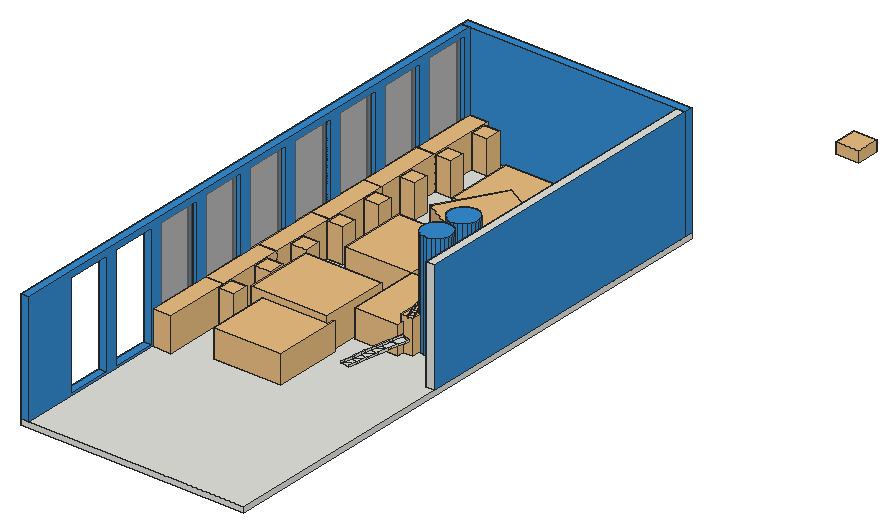
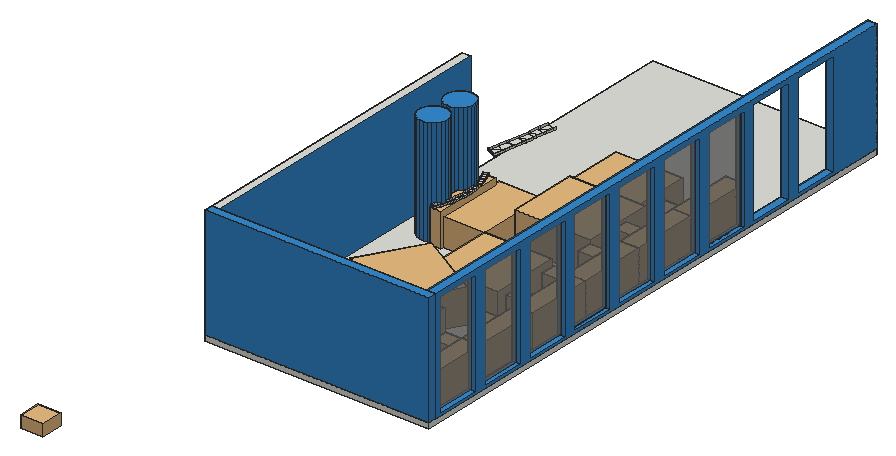
# SketchUp Ruby script. Lengths in inches.
U = 1.inch
M = Sketchup.active_model
def pt(a) = Geom::Point3d.new(a.map { |v| v * U })
def face(e, loops, mat)
  f = e.add_face(loops[0].map { |a| pt(a) })
  loops[1..].each { |l| e.add_face(l.map { |a| pt(a) }).erase! }
  f.material = f.back_material = mat if mat
  f
end
# faces: each face lists its corners as indices into pts; further lists are holes
def faces(e, pts, list, mat = nil) = list.each { |f| face(e, (f[0].is_a?(Array) ? f : [f]).map { |l| l.map { |i| pts[i] } }, mat) }
# xy, xz, yz: faces in a plane at the given z, y or x. An outline is a flat list of corners, or four numbers for a rectangle; further outlines are holes
def ring(l) = l.size == 4 ? [[l[0], l[1]], [l[2], l[1]], [l[2], l[3]], [l[0], l[3]]] : l.each_slice(2).to_a
def flat(e, list, mat, &to3) = list.each { |f| face(e, (f[0].is_a?(Array) ? f : [f]).map { |l| ring(l).map { |u, v| to3.(u, v) } }, mat) }
def xy(e, z, list, mat = nil) = flat(e, list, mat) { |x, y| [x, y, z] }
def xz(e, y, list, mat = nil) = flat(e, list, mat) { |x, z| [x, y, z] }
def yz(e, x, list, mat = nil) = flat(e, list, mat) { |y, z| [x, y, z] }
def lines(e, pts, list) = list.each { |a, b| e.add_line(pt(pts[a]), pt(pts[b])) }
# prism: a flat outline (further loops are holes) pulled along v
def prism(e, loops, v, mat = nil)
  f = face(e, loops, mat); d = Geom::Vector3d.new(v.map { |x| x * U })
  f.pushpull(f.normal.samedirection?(d) ? d.length : -d.length)
end
def box(e, o, s, mat = nil) = prism(e, [[o, [o[0] + s[0], o[1], o[2]], [o[0] + s[0], o[1] + s[1], o[2]], [o[0], o[1] + s[1], o[2]]]], [0, 0, s[2]], mat)
def at(x, y, z, deg = 0) = Geom::Transformation.translation(pt([x, y, z])) * Geom::Transformation.rotation(ORIGIN, Z_AXIS, deg.degrees)
def axes(o, x, y, z) = Geom::Transformation.new([*x, 0, *y, 0, *z, 0, *pt(o).to_a, 1])
def part(name) = M.definitions.add(name)
# library, detail: a bought-in or finely detailed component or shape, given as its bounding box
def library(name, o, s) = part(name).tap { |d| box(d.entities, o, s) }
def detail(e, o, s) = box(e.add_group.entities, o, s)
def put(e, d, t, mat = nil) = e.add_instance(d, t).tap { |i| i.material = mat if mat }
def group(e, t, mat = nil) = e.add_group.tap { |g| g.transformation = t; g.material = mat if mat }.entities
root = M.entities
M.materials.add("[Color I07]").color = [53, 140, 209]
M.materials.add("[Mirror 01]").color = [185, 185, 185]
M.materials.add("[Translucent Glass Gray]").color = [128, 128, 128]
M.materials["[Translucent Glass Gray]"].alpha = 0.5
c1 = library("Edge Console",[-35.43,-9.84,0],[70.86,19.68,29.53])
c2 = library("MARBLE DINING TABLE",[-16.8,-22.21,-0.08],[92.52,94.06,29.61])
c3 = library("Group\#15",[-0.03,0,0],[16.43,16.29,39.54])
c4 = part("Group\#10")
detail(c4.entities,[-4.72,-9.03,0],[81.56,73.05,36])
c5 = library("MARBLE DINING TABLE\#1",[-8.71,-22.21,-0.08],[73.21,94.06,29.61])
c6 = library("Group\#7",[-0.48,-8.49,0],[72.96,12.49,36])
c7 = part("Group\#2")
box(c7.entities,[0,0,0],[240,9,120])
c8 = library("Dome Light",[-12,-12,0],[24,24,12])
box(root,[4.25,237.22,8],[0.5,48,112],"[Translucent Glass Gray]")
box(root,[4.25,297.22,8],[0.5,48,112],"[Translucent Glass Gray]")
box(root,[4.25,417.22,8],[0.5,48,112],"[Translucent Glass Gray]")
box(root,[4.25,477.22,8],[0.5,48,112],"[Translucent Glass Gray]")
box(root,[4.25,537.22,8],[0.5,48,112],"[Translucent Glass Gray]")
xy(root,6,[[0,0.22,9,591.22],[231.01,255.46,240,591.22]])
xy(root,8,[[4.25,177.22,4.75,225.22],[4.25,357.22,4.75,405.22]])
xy(root,42,[[200.12,191.2,191.15,192.67,191.71,196.1,201.35,199.47],[191.15,192.67,190.16,192.8,190.72,196.23,191.71,196.1],[191.71,196.1,190.72,196.23,191.59,203.74,192.58,203.59],[191.71,196.1,192.58,203.59,201.57,201.74,201.35,199.47],[201.57,201.74,192.58,203.59,193.2,207.06,203.09,211.07],
  [192.58,203.59,191.59,203.74,192.21,207.21,193.2,207.06],[193.2,207.06,192.21,207.21,193.21,214.83,194.2,214.68],[193.2,207.06,194.2,214.68,203.24,212.39,203.09,211.07],[203.24,212.39,194.2,214.68,194.97,218.73,204.76,223.26,205.13,223.13],[194.2,214.68,193.21,214.83,193.99,218.9,194.97,218.73],
  [194.97,218.73,193.99,218.9,195.01,226.07,196,225.9],[194.97,218.73,196,225.9,204.76,223.26],[205.13,223.13,204.76,223.26,205.21,223.47],[204.76,223.26,196,225.9,197.09,231.29,204.28,235.05,207.19,233.91,205.21,223.47],[196,225.9,195.01,226.07,196.1,231.47,197.09,231.29],
  [197.09,231.29,196.1,231.47,197.03,237.42,198.01,237.24],[197.09,231.29,198.01,237.24,204.28,235.05],[207.19,233.91,204.28,235.05,207.95,236.97],[204.28,235.05,198.01,237.24,199.65,244.98,203.64,247.3125,209.51,244.7,207.95,236.97],[198.01,237.24,197.03,237.42,198.66,245.16,199.65,244.98],
  [209.51,244.7,203.64,247.3125,211.37,251.84],[199.65,244.98,198.66,245.16,199.28,248.84,200.26,248.65],[199.65,244.98,200.26,248.65,203.64,247.3125],[203.64,247.3125,200.26,248.65,202.8,260.09,212.15,255.46,211.37,251.84],[200.26,248.65,199.28,248.84,201.82,260.31,202.8,260.09],
  [185.34,288.6,183.92,291.45,184.83,291.875,186.23,289.04],[186.23,289.04,184.83,291.875,188.44,293.58,189.78,290.89],[183.92,291.45,182.61,294.37,183.54,294.76,184.83,291.875],[184.83,291.875,183.54,294.76,187.22,296.32,188.44,293.58],[182.61,294.37,181.42,297.34,182.36,297.69,183.54,294.76],
  [183.54,294.76,182.36,297.69,186.1,299.1,187.22,296.32],[181.42,297.34,180.36,300.35,181.3,300.67,182.36,297.69],[182.36,297.69,181.3,300.67,185.1,301.93,186.1,299.1],[180.36,300.35,179.41,303.41,180.37,303.6875,181.3,300.67],[181.3,300.67,180.37,303.6875,184.21,304.8,185.1,301.93],
  [179.41,303.41,178.58,306.5,179.55,306.74,180.37,303.6875],[180.37,303.6875,179.55,306.74,183.44,307.69,184.21,304.8],[178.58,306.5,177.88,309.625,178.86,309.83,179.55,306.74],[179.55,306.74,178.86,309.83,182.78,310.62,183.44,307.69],[177.88,309.625,177.31,312.77,178.3,312.93,178.86,309.83],
  [178.86,309.83,178.3,312.93,182.25,313.57,182.78,310.62],[177.31,312.77,176.86,315.94,177.85,316.0625,178.3,312.93],[178.3,312.93,177.85,316.0625,181.83,316.54,182.25,313.57],[176.86,315.94,176.54,319.13,177.54,319.21,177.85,316.0625],[177.85,316.0625,177.54,319.21,181.53,319.53,181.83,316.54],
  [176.54,319.13,176.35,322.32,177.35,322.36,177.54,319.21],[177.54,319.21,177.35,322.36,181.35,322.52,181.53,319.53],[176.35,322.32,176.29,325.52,177.29,325.52,177.35,322.36],[177.35,322.36,177.29,325.52,181.29,325.52,181.35,322.52],[176.29,325.52,176.35,328.72,177.35,328.68,177.29,325.52],
  [177.29,325.52,177.35,328.68,181.35,328.52,181.29,325.52],[181.35,328.52,177.35,328.68,177.54,331.84,181.53,331.52],[177.35,328.68,176.35,328.72,176.54,331.92,177.54,331.84],[181.53,331.52,177.54,331.84,177.85,334.98,181.83,334.5],[177.54,331.84,176.54,331.92,176.86,335.1,177.85,334.98],
  [181.83,334.5,177.85,334.98,178.3,338.11,182.25,337.47],[177.85,334.98,176.86,335.1,177.31,338.27,178.3,338.11],[182.25,337.47,178.3,338.11,178.86,341.22,182.78,340.42],[178.3,338.11,177.31,338.27,177.88,341.42,178.86,341.22],[182.78,340.42,178.86,341.22,179.55,344.3,183.44,343.35],
  [178.86,341.22,177.88,341.42,178.58,344.54,179.55,344.3],[183.44,343.35,179.55,344.3,180.37,347.35,184.21,346.25],[179.55,344.3,178.58,344.54,179.41,347.63,180.37,347.35],[184.21,346.25,180.37,347.35,181.3,350.375,185.1,349.11],[180.37,347.35,179.41,347.63,180.36,350.6875,181.3,350.375],
  [185.1,349.11,181.3,350.375,182.36,353.35,186.1,351.94],[181.3,350.375,180.36,350.6875,181.42,353.7,182.36,353.35],[186.1,351.94,182.36,353.35,183.54,356.29,187.22,354.72],[182.36,353.35,181.42,353.7,182.61,356.68,183.54,356.29],[187.22,354.72,183.54,356.29,184.83,359.17,188.44,357.46],
  [183.54,356.29,182.61,356.68,183.92,359.6,184.83,359.17],[188.44,357.46,184.83,359.17,186.23,362,189.78,360.15],[184.83,359.17,183.92,359.6,185.34,362.44,186.23,362]])
xy(root,120,[[4.25,177.22,4.75,225.22],[4.25,357.22,4.75,405.22]])
xy(root,126,[[231.01,255.46,240,591.22]])
xz(root,177.22,[[4.25,8,4.75,120]])
xz(root,225.22,[[4.25,8,4.75,120]])
xz(root,255.46,[[231.01,6,240,126]])
xz(root,357.22,[[4.25,8,4.75,120]])
xz(root,405.22,[[4.25,8,4.75,120]])
xz(root,591.22,[[0,6,9,126],[231.01,6,240,126]])
yz(root,4.25,[[177.22,8,225.22,120],[357.22,8,405.22,120]],"[Translucent Glass Gray]")
yz(root,4.75,[[177.22,8,225.22,120],[357.22,8,405.22,120]],"[Translucent Glass Gray]")
yz(root,231.01,[[255.46,6,591.22,126]],"[Color I07]")
yz(root,240,[[255.46,6,591.22,126]],"[Color I07]")
p = [[201.35,199.47,42],[201.35,199.47,44],[200.12,191.2,44],[200.12,191.2,42],[190.16,192.8,44],[190.72,196.23,44],
  [190.72,196.23,42],[190.16,192.8,42],[191.71,196.1,44],[191.71,196.1,42],[192.58,203.59,42],[192.58,203.59,44],
  [191.59,203.74,44],[191.59,203.74,42],[201.57,201.74,42],[201.57,201.74,44],[203.09,211.07,42],[203.09,211.07,44],
  [193.2,207.06,42],[193.2,207.06,44],[192.21,207.21,44],[192.21,207.21,42],[194.2,214.68,42],[194.2,214.68,44],
  [193.21,214.83,44],[193.21,214.83,42],[203.24,212.39,42],[203.24,212.39,44],[205.13,223.13,42],[205.13,223.13,44],
  [194.97,218.73,42],[194.97,218.73,44],[193.99,218.9,44],[193.99,218.9,42],[196,225.9,42],[196,225.9,44],
  [195.01,226.07,44],[195.01,226.07,42],[205.21,223.47,42],[205.21,223.47,44],[207.19,233.91,42],[207.19,233.91,44],
  [197.09,231.29,42],[197.09,231.29,44],[196.1,231.47,44],[196.1,231.47,42],[198.01,237.24,42],[198.01,237.24,44],
  [197.03,237.42,44],[197.03,237.42,42],[207.95,236.97,42],[207.95,236.97,44],[209.51,244.7,42],[209.51,244.7,44],
  [199.65,244.98,42],[199.65,244.98,44],[198.66,245.16,44],[198.66,245.16,42],[211.37,251.84,42],[211.37,251.84,44],
  [200.26,248.65,42],[200.26,248.65,44],[199.28,248.84,44],[199.28,248.84,42],[202.8,260.09,42],[202.8,260.09,44],
  [201.82,260.31,44],[201.82,260.31,42],[212.15,255.46,42],[212.15,255.46,44],[185.34,288.6,44],[183.92,291.45,44],
  [183.92,291.45,42],[185.34,288.6,42],[186.23,289.04,44],[186.23,289.04,42],[189.78,290.89,42],[189.78,290.89,44],
  [188.44,293.58,42],[188.44,293.58,44],[182.61,294.37,44],[182.61,294.37,42],[187.22,296.32,42],[187.22,296.32,44],
  [181.42,297.34,44],[181.42,297.34,42],[186.1,299.1,42],[186.1,299.1,44],[180.36,300.35,44],[180.36,300.35,42],
  [185.1,301.93,42],[185.1,301.93,44],[179.41,303.41,44],[179.41,303.41,42],[184.21,304.8,42],[184.21,304.8,44],
  [178.58,306.5,44],[178.58,306.5,42],[183.44,307.69,42],[183.44,307.69,44],[177.88,309.625,44],[177.88,309.625,42],
  [182.78,310.62,42],[182.78,310.62,44],[177.31,312.77,44],[177.31,312.77,42],[182.25,313.57,42],[182.25,313.57,44],
  [176.86,315.94,44],[176.86,315.94,42],[181.83,316.54,42],[181.83,316.54,44],[176.54,319.13,44],[176.54,319.13,42],
  [181.53,319.53,42],[181.53,319.53,44],[176.35,322.32,44],[176.35,322.32,42],[181.35,322.52,42],[181.35,322.52,44],
  [176.29,325.52,44],[176.29,325.52,42],[181.29,325.52,42],[181.29,325.52,44],[176.35,328.72,44],[176.35,328.72,42],
  [181.35,328.52,42],[181.35,328.52,44],[181.53,331.52,42],[181.53,331.52,44],[176.54,331.92,44],[176.54,331.92,42],
  [181.83,334.5,42],[181.83,334.5,44],[176.86,335.1,44],[176.86,335.1,42],[182.25,337.47,42],[182.25,337.47,44],
  [177.31,338.27,44],[177.31,338.27,42],[182.78,340.42,42],[182.78,340.42,44],[177.88,341.42,44],[177.88,341.42,42],
  [183.44,343.35,42],[183.44,343.35,44],[178.58,344.54,44],[178.58,344.54,42],[184.21,346.25,42],[184.21,346.25,44],
  [179.41,347.63,44],[179.41,347.63,42],[185.1,349.11,42],[185.1,349.11,44],[180.36,350.6875,44],[180.36,350.6875,42],
  [186.1,351.94,42],[186.1,351.94,44],[181.42,353.7,44],[181.42,353.7,42],[187.22,354.72,42],[187.22,354.72,44],
  [182.61,356.68,44],[182.61,356.68,42],[188.44,357.46,42],[188.44,357.46,44],[183.92,359.6,44],[183.92,359.6,42],
  [189.78,360.15,42],[189.78,360.15,44],[185.34,362.44,44],[185.34,362.44,42],[186.23,362,42],[186.23,362,44]]
faces(root,p,[[0,1,2,3],[4,5,6,7],[8,9,10,11],[5,12,13,6],[14,15,1,0],[16,17,15,14],[11,10,18,19],[12,20,21,13],
  [19,18,22,23],[20,24,25,21],[26,27,17,16],[28,29,27,26],[23,22,30,31],[24,32,33,25],[31,30,34,35],[32,36,37,33],
  [38,39,29,28],[40,41,39,38],[35,34,42,43],[36,44,45,37],[43,42,46,47],[44,48,49,45],[50,51,41,40],[52,53,51,50],
  [47,46,54,55],[48,56,57,49],[58,59,53,52],[55,54,60,61],[56,62,63,57],[61,60,64,65],[62,66,67,63],[68,69,59,58],
  [64,65,69,68],[64,67,66,65],[70,71,72,73],[74,70,73,75],[76,77,74,75],[78,79,77,76],[71,80,81,72],[82,83,79,78],
  [80,84,85,81],[86,87,83,82],[84,88,89,85],[90,91,87,86],[88,92,93,89],[94,95,91,90],[92,96,97,93],[98,99,95,94],
  [96,100,101,97],[102,103,99,98],[100,104,105,101],[106,107,103,102],[104,108,109,105],[110,111,107,106],[108,112,113,109],[114,115,111,110],
  [112,116,117,113],[118,119,115,114],[116,120,121,117],[122,123,119,118],[120,124,125,121],[126,127,123,122],[128,129,127,126],[124,130,131,125],
  [132,133,129,128],[130,134,135,131],[136,137,133,132],[134,138,139,135],[140,141,137,136],[138,142,143,139],[144,145,141,140],[142,146,147,143],
  [148,149,145,144],[146,150,151,147],[152,153,149,148],[150,154,155,151],[156,157,153,152],[154,158,159,155],[160,161,157,156],[158,162,163,159],
  [164,165,161,160],[162,166,167,163],[168,169,165,164],[166,170,171,167],[172,173,169,168],[172,171,170,173]])
put(root,c1,axes([18.84,201.77,6],[0,1,0],[-1,0,0],[0,0,1.21911]))
put(root,c2,axes([74.9375,199.02,6.08],[0.77821,0,0],[0,0.76543,0],[0,0,1]))
put(root,c3,axes([29.5,229.65,6],[1,0,0],[0,1,0],[0,0,0.902]))
put(root,c1,axes([18.84,272.56,6],[0,1,0],[-1,0,0],[0,0,1.21911]))
put(root,c4,at(54.24,257.01,6),"[Mirror 01]")
put(root,c3,axes([29.5,278.12,6],[1,0,0],[0,1,0],[0,0,0.902]))
g1 = group(root,at(0,0.22,6),"[Color I07]")
prism(g1,[[[0,591,0],[0,0,0],[0,0,120],[0,591,120]],[[0,537,114],[0,537,2],[0,585,2],[0,585,114]],[[0,477,114],[0,477,2],[0,525,2],[0,525,114]],[[0,417,114],[0,417,2],[0,465,2],[0,465,114]],[[0,357,114],[0,357,2],[0,405,2],[0,405,114]],[[0,297,114],[0,297,2],[0,345,2],[0,345,114]],[[0,237,114],[0,237,2],[0,285,2],[0,285,114]],[[0,177,114],[0,177,2],[0,225,2],[0,225,114]],[[0,117,114],[0,117,2],[0,165,2],[0,165,114]],[[0,57,114],[0,57,2],[0,105,2],[0,105,114]]],[9,0,0])
g2 = group(root,at(0,0.22,0))
box(g2,[0,0,0],[240,600,6])
g3 = group(root,at(182.92,296.19,6),"[Color I07]")
prism(g3,[[[30.12,12.82,0],[29.01,9.01,0],[26.96,5.61,0],[24.11,2.87,0],[20.63,0.95,0],[16.78,0,0],[12.82,0.08,0],[9.01,1.18,0],[5.61,3.23,0],[2.87,6.09,0],[0.95,9.56,0],[0,13.41,0],[0.08,17.375,0],[1.18,21.18,0],[3.23,24.58,0],[6.09,27.33,0],[9.56,29.24,0],[13.41,30.19,0],[17.375,30.12,0],[21.18,29.01,0],[24.58,26.96,0],[27.33,24.11,0],[29.24,20.63,0],[30.19,16.78,0]]],[0,0,114.1875])
put(root,c5,axes([138.35,300.37,6.08],[0.63,0,0],[0,0.82,0],[0,0,1]))
put(root,c6,at(181.29,289.52,6,90),"[Color I07]")
put(root,c3,axes([29.5,326.59,6],[1,0,0],[0,1,0],[0,0,0.902]))
put(root,c1,axes([18.84,343.36,6],[0,1,0],[-1,0,0],[0,0,1.21911]))
g4 = group(root,at(184.43,330.14,6),"[Color I07]")
prism(g4,[[[30.12,12.82,0],[29.01,9.01,0],[26.96,5.61,0],[24.11,2.87,0],[20.63,0.95,0],[16.78,0,0],[12.82,0.08,0],[9.01,1.18,0],[5.61,3.23,0],[2.87,6.09,0],[0.95,9.56,0],[0,13.41,0],[0.08,17.375,0],[1.18,21.18,0],[3.23,24.58,0],[6.09,27.33,0],[9.56,29.24,0],[13.41,30.19,0],[17.375,30.12,0],[21.18,29.01,0],[24.58,26.96,0],[27.33,24.11,0],[29.24,20.63,0],[30.19,16.78,0]]],[0,0,114.1875])
put(root,c3,axes([29.5,375.06,6],[1,0,0],[0,1,0],[0,0,0.902]))
put(root,c2,axes([74.9375,375.46,6.08],[0.77821,0,0],[0,0.76543,0],[0,0,1]))
put(root,c1,axes([18.84,414.1875,6],[0,1,0],[-1,0,0],[0,0,1.21911]))
put(root,c3,axes([29.5,423.53,6],[1,0,0],[0,1,0],[0,0,0.902]))
put(root,c4,at(88.62,455.13,6,-30),"[Mirror 01]")
put(root,c3,axes([29.5,472,6],[1,0,0],[0,1,0],[0,0,0.902]))
put(root,c1,axes([18.84,484.95,6],[0,1,0],[-1,0,0],[0,0,1.21911]))
put(root,c2,axes([92.39,497.13,6.08],[0.77821,0,0],[0,0.76543,0],[0,0,1]))
put(root,c3,axes([29.5,520.47,6],[1,0,0],[0,1,0],[0,0,0.902]))
put(root,c1,axes([18.84,555.78,6],[0,1,0],[-1,0,0],[0,0,1.21911]))
put(root,c3,axes([29.5,568.95,6],[1,0,0],[0,1,0],[0,0,0.902]))
put(root,c7,at(0,591.22,6),"[Color I07]")
put(root,c8,at(256.33,800.68,0))
